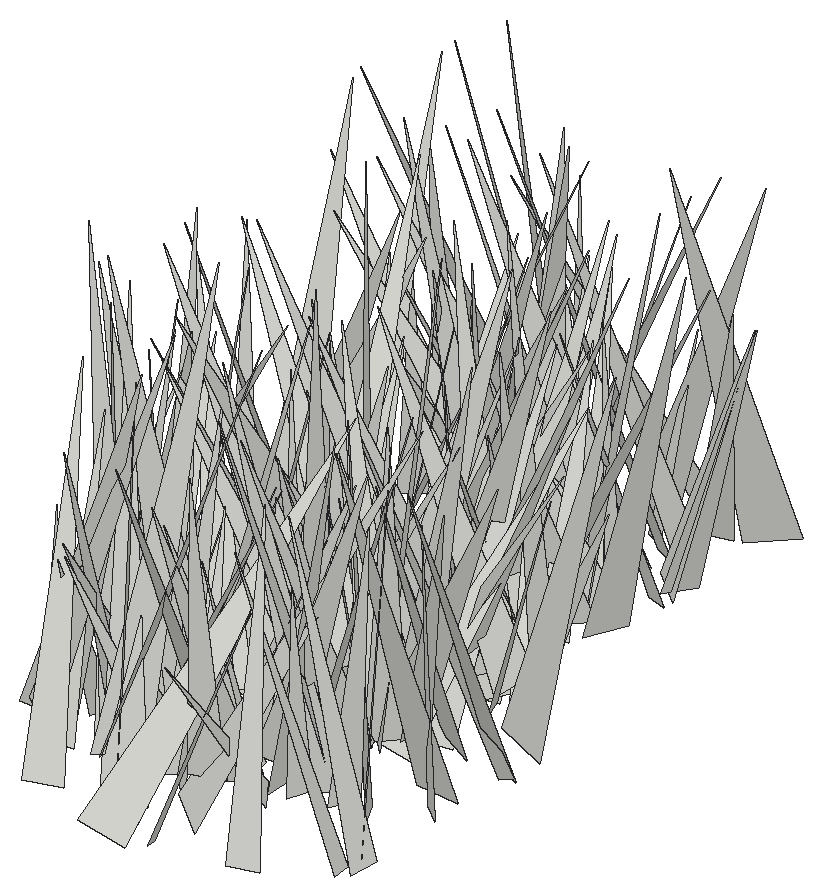
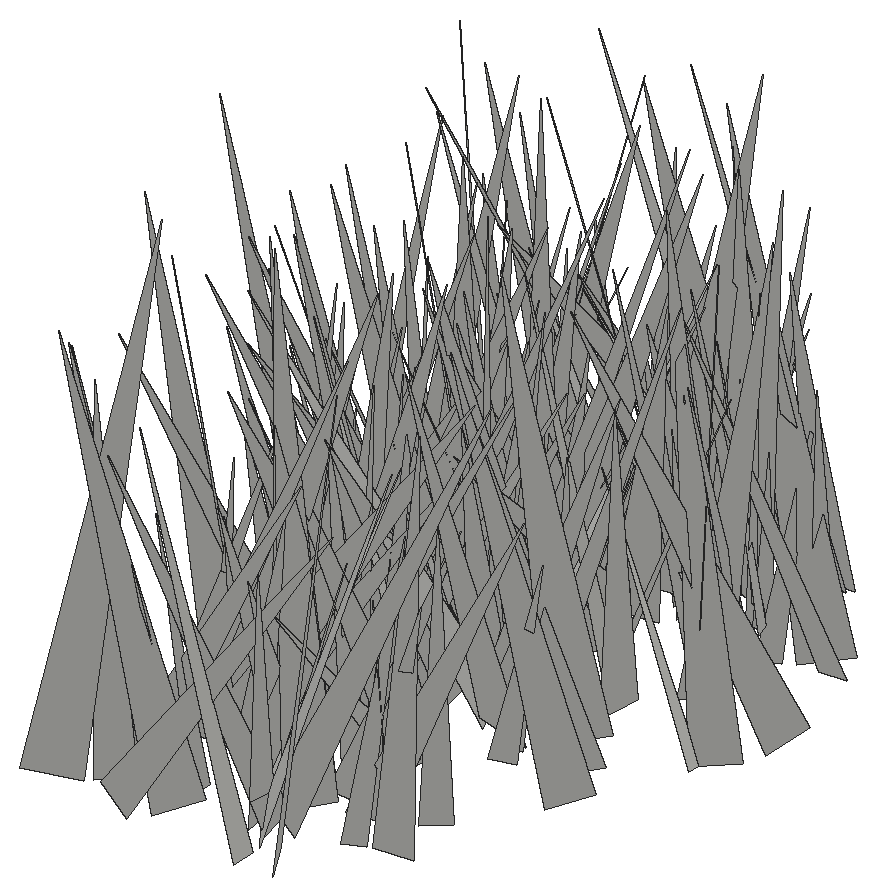
# SketchUp Ruby script. Lengths in inches.
U = 1.inch
M = Sketchup.active_model
def pt(a) = Geom::Point3d.new(a.map { |v| v * U })
def face(e, loops, mat)
  f = e.add_face(loops[0].map { |a| pt(a) })
  loops[1..].each { |l| e.add_face(l.map { |a| pt(a) }).erase! }
  f.material = f.back_material = mat if mat
  f
end
# faces: each face lists its corners as indices into pts; further lists are holes
def faces(e, pts, list, mat = nil) = list.each { |f| face(e, (f[0].is_a?(Array) ? f : [f]).map { |l| l.map { |i| pts[i] } }, mat) }
# xy, xz, yz: faces in a plane at the given z, y or x. An outline is a flat list of corners, or four numbers for a rectangle; further outlines are holes
def ring(l) = l.size == 4 ? [[l[0], l[1]], [l[2], l[1]], [l[2], l[3]], [l[0], l[3]]] : l.each_slice(2).to_a
def flat(e, list, mat, &to3) = list.each { |f| face(e, (f[0].is_a?(Array) ? f : [f]).map { |l| ring(l).map { |u, v| to3.(u, v) } }, mat) }
def xy(e, z, list, mat = nil) = flat(e, list, mat) { |x, y| [x, y, z] }
def xz(e, y, list, mat = nil) = flat(e, list, mat) { |x, z| [x, y, z] }
def yz(e, x, list, mat = nil) = flat(e, list, mat) { |y, z| [x, y, z] }
def lines(e, pts, list) = list.each { |a, b| e.add_line(pt(pts[a]), pt(pts[b])) }
# prism: a flat outline (further loops are holes) pulled along v
def prism(e, loops, v, mat = nil)
  f = face(e, loops, mat); d = Geom::Vector3d.new(v.map { |x| x * U })
  f.pushpull(f.normal.samedirection?(d) ? d.length : -d.length)
end
def box(e, o, s, mat = nil) = prism(e, [[o, [o[0] + s[0], o[1], o[2]], [o[0] + s[0], o[1] + s[1], o[2]], [o[0], o[1] + s[1], o[2]]]], [0, 0, s[2]], mat)
def at(x, y, z, deg = 0) = Geom::Transformation.translation(pt([x, y, z])) * Geom::Transformation.rotation(ORIGIN, Z_AXIS, deg.degrees)
def axes(o, x, y, z) = Geom::Transformation.new([*x, 0, *y, 0, *z, 0, *pt(o).to_a, 1])
def part(name) = M.definitions.add(name)
# library, detail: a bought-in or finely detailed component or shape, given as its bounding box
def library(name, o, s) = part(name).tap { |d| box(d.entities, o, s) }
def detail(e, o, s) = box(e.add_group.entities, o, s)
def put(e, d, t, mat = nil) = e.add_instance(d, t).tap { |i| i.material = mat if mat }
def group(e, t, mat = nil) = e.add_group.tap { |g| g.transformation = t; g.material = mat if mat }.entities
root = M.entities
c1 = part("fur_instance\#9")
p = [[0.8125,0,1.79],[0.67,-0.02,1.48],[0,-0.11,0],[0,0.11,0]]
faces(c1.entities,p,[[0,1,2,3]])
put(root,c1,axes([148.45,197.79,-28.22],[4.8815,3.3845,2.02519],[2.72156,-5.22275,2.16824],[-2.85471,0.80828,5.53015]))
put(root,c1,axes([148.84,203.19,-27.1],[-5.6137,1.8249,1.28834],[1.63706,5.7317,-0.98561],[1.51991,0.56669,5.82001]))
put(root,c1,axes([148.67,199.6,-28.22],[-6.28621,2.90163,2.83322],[3.4688,6.55463,0.9835],[2.10096,-2.14018,6.85337]))
put(root,c1,axes([150.45,212.51,-27.1],[-4.33976,4.07233,1.17149],[4.17045,3.80756,2.21352],[-0.75076,-2.38923,5.52429]))
put(root,c1,axes([148.03,194.95,-28.22],[-3.33469,1.40616,1.82105],[1.56398,3.73727,-0.02186],[1.68745,-0.685,3.61897]))
put(root,c1,axes([145.95,202.4375,-28.22],[2.99312,-6.69994,0.30324],[-6.59145,-2.87731,1.48788],[1.23852,0.87852,7.18569]))
put(root,c1,axes([146.57,196.35,-28.22],[1.84734,5.85191,0.92453],[5.8229,-1.61485,-1.41361],[1.09242,-1.28828,5.97153]))
put(root,c1,axes([146.28,202.97,-28.22],[4.26627,1.55205,0.05399],[1.49304,-4.05567,-1.39111],[0.42732,-1.32496,4.32143]))
put(root,c1,axes([145.1875,200.12,-28.22],[6.82569,-2.14516,0.01525],[-2.06759,-6.56497,1.95405],[0.57187,1.86856,6.88284]))
put(root,c1,axes([147.71,200.6,-28.22],[0.28341,4.29415,2.46111],[4.89058,0.13603,-0.80051],[0.76092,-2.47364,4.22839]))
put(root,c1,axes([149.52,207.61,-27.1],[-2.08975,2.94897,0.92989],[3.09202,1.98432,0.65582],[-0.0238,-1.13764,3.55435]))
put(root,c1,axes([150.25,195.58,-27.1],[-7.50799,1.69583,1.59774],[1.55933,7.66276,-0.80567],[1.73121,0.45255,7.65484]))
put(root,c1,axes([150.14,195.61,-28.22],[-6.12572,-2.31991,2.2614],[-2.97153,5.95041,-1.94497],[1.2907,2.68904,6.25488]))
put(root,c1,axes([148.5,196.86,-28.22],[3.04717,-2.22298,0.43436],[-2.028,-3.00193,-1.13631],[-1.00873,-0.67996,3.59662]))
put(root,c1,axes([148.62,213.68,-27.1],[0.4786,-6.17329,1.68247],[-6.39725,-0.42884,0.2463],[0.12453,1.69584,6.18692]))
put(root,c1,axes([150.45,204.91,-27.1],[-3.80657,-5.75041,0.9295],[-5.82495,3.76407,-0.56819],[0.03325,1.08891,6.87272]))
put(root,c1,axes([148.57,205.27,-27.1],[-4.94866,6.16749,2.69055],[6.18584,5.48419,-1.19385],[2.6481,-1.28527,7.81677]))
put(root,c1,axes([149.66,195.58,-28.22],[-0.46969,3.55211,0.73396],[3.59032,0.35011,0.60316],[-0.51554,-0.79795,3.53189]))
put(root,c1,axes([146.56,208.22,-27.1],[5.35038,-4.23141,0.69897],[-4.27634,-5.17862,1.38378],[0.32603,1.51562,6.67957]))
put(root,c1,axes([149.92,192.2,-28.22],[-1.0825,6.58238,0.66021],[6.6005,1.02978,0.55528],[-0.44383,-0.73975,6.64764]))
put(root,c1,axes([151.19,205.61,-27.1],[-5.49496,2.98551,0.84144],[3.09795,5.36781,1.18541],[0.15494,-1.44541,6.14025]))
put(root,c1,axes([148.7,211.6,-27.1],[2.93376,-3.22318,1.07266],[-3.3076,-3.03341,-0.06853],[-0.77414,0.74566,4.35788]))
put(root,c1,axes([149.74,202.73,-27.1],[-4.13984,-2.04423,0.54277],[-1.65039,3.86825,1.98107],[1.32277,-1.57147,4.17043]))
put(root,c1,axes([151.35,210.93,-27.1],[-1.53438,4.71255,0.03454],[4.47921,1.44703,1.55125],[-1.46492,-0.51147,4.70702]))
put(root,c1,axes([148.5,197.11,-27.1],[3.90059,1.73334,0.99556],[1.91928,-3.85762,-0.80331],[-0.55855,-1.15086,4.19211]))
put(root,c1,axes([152.39,214.02,-27.1],[-3.30387,-7.05223,0.96215],[-6.92829,2.9435,-2.21582],[-1.63048,1.78244,7.4659]))
put(root,c1,axes([150,192.89,-27.1],[0.07202,5.27236,0.64208],[5.29211,-0.12578,0.43929],[-0.45123,-0.63374,5.25452]))
put(root,c1,axes([149.73,196.04,-27.1],[1.82838,5.64567,1.15342],[5.69001,-1.95997,0.57384],[-0.90985,-0.91206,5.90655]))
put(root,c1,axes([150.57,206.29,-27.1],[0.71123,8.26754,0.30404],[8.18462,-0.74766,1.1847],[-1.20692,-0.19821,8.21307]))
put(root,c1,axes([152.47,214.85,-27.1],[-6.0406,-4.0795,1.11122],[-4.22494,5.74856,-1.86274],[-0.16426,2.16279,7.04708]))
put(root,c1,axes([149.84,206.84,-27.1],[0.38747,-3.62863,0.53891],[-3.66751,-0.39531,-0.02484],[-0.08219,0.53319,3.64917]))
put(root,c1,axes([150.79,197.07,-27.1],[-7.20595,2.28011,2.02761],[1.9171,7.42879,-1.54068],[2.37378,0.922,7.39939]))
put(root,c1,axes([150.32,197.63,-27.1],[-4.40906,-3.22075,2.19411],[-3.50304,4.72714,-0.10035],[1.70765,1.38134,5.45921]))
put(root,c1,axes([151.9,198.71,-27.1],[-2.77056,6.19265,0.76015],[6.19361,2.62958,1.15202],[-0.75223,-1.15721,6.68563]))
put(root,c1,axes([147.24,195.79,-28.22],[3.43501,-7.39782,1.03394],[-7.28345,-3.06455,2.27067],[1.65774,1.86463,7.83397]))
put(root,c1,axes([150.1,212.05,-27.1],[-2.43911,-2.15453,1.73505],[-2.51562,2.68975,-0.19638],[1.15067,1.31336,3.24849]))
put(root,c1,axes([150.4,196.83,-27.1],[-3.17134,4.85922,0.78552],[4.77597,3.26378,-0.90795],[1.19131,-0.14895,5.73106]))
put(root,c1,axes([150.9,216.07,-27.1],[-6.29622,-3.82649,2.40942],[-4.00808,6.63484,0.06324],[2.09347,1.19444,7.36752]))
put(root,c1,axes([149.81,213.97,-27.1],[4.21418,-1.38432,0.79636],[-0.98829,-4.02576,-1.76817],[-1.25452,-1.47878,4.06808]))
put(root,c1,axes([150.43,197.78,-28.22],[6.05789,3.57549,2.196],[3.19122,-6.43003,1.66595],[-2.72445,0.41853,6.83424]))
put(root,c1,axes([147.38,206.58,-27.1],[1.67696,-6.87357,2.26471],[-6.67493,-0.57073,3.21041],[2.79647,2.7596,6.30488]))
put(root,c1,axes([150.59,197.1,-28.22],[3.46816,-3.92613,0.03464],[-3.68547,-3.27126,-1.77763],[-1.35388,-1.15247,4.92774]))
put(root,c1,axes([150.375,196.96,-28.22],[3.62249,2.81644,0.55831],[2.6251,-3.61284,1.19278],[-1.16313,0.61769,4.43081]))
put(root,c1,axes([150.95,194.77,-27.1],[-1.08369,-5.40972,1.03151],[-5.49173,1.14023,0.21038],[0.41232,0.96864,5.51318]))
put(root,c1,axes([153.38,213.62,-27.1],[-5.70122,-3.26457,0.62497],[-3.32356,5.6155,-0.98593],[0.04408,1.16649,6.49533]))
put(root,c1,axes([148.5,193.81,-27.1],[4.58596,6.39713,1.96066],[6.63658,-4.04695,-2.31874],[0.85046,-2.91504,7.52182]))
put(root,c1,axes([152.2,201.56,-27.1],[0.68638,4.30492,0.85677],[4.11958,-0.93113,1.37825],[-1.51508,-0.58153,4.13569]))
put(root,c1,axes([152.6,192.77,-28.22],[-0.59735,8.07244,1.41711],[8.08686,0.34954,1.4177],[-1.33238,-1.49761,7.96939]))
put(root,c1,axes([152.82,202.95,-28.22],[-5.31992,-4.92486,0.01845],[-4.88394,5.27914,0.91325],[0.63384,-0.65774,7.19179]))
put(root,c1,axes([152.01,197.05,-27.1],[2.92408,-7.38877,2.72238],[-7.56214,-3.44459,-1.22649],[-2.19528,2.02396,7.85111]))
put(root,c1,axes([151.8,211.95,-27.1],[1.73038,-3.85975,0.19684],[-3.59553,-1.68683,-1.46882],[-1.41726,-0.43309,3.96667]))
put(root,c1,axes([150.76,204,-27.1],[2.98723,-2.64764,1.00912],[-2.72025,-3.09017,-0.05514],[-0.79284,0.62671,3.99131]))
put(root,c1,axes([152.11,194.84,-27.1],[-3.71284,-0.24914,0.82183],[0.046,3.58403,1.29433],[0.85753,-1.27095,3.48884]))
put(root,c1,axes([153.27,201.42,-27.1],[-6.87965,3.10007,2.46286],[3.78941,6.58637,2.29475],[1.14737,-3.16466,7.18848]))
put(root,c1,axes([153.77,200.68,-27.1],[-5.93019,0.58333,0.46706],[0.68124,5.75556,1.46115],[0.30714,-1.50292,5.77689]))
put(root,c1,axes([154.13,210.92,-27.1],[-6.77007,0.71674,0.61078],[0.8862,6.3486,2.37288],[0.31848,-2.42944,6.38099]))
put(root,c1,axes([151.22,194.29,-28.22],[5.6621,3.46946,2.68851],[3.90579,-5.98471,-0.5026],[-2.00251,-1.86297,6.62147]))
put(root,c1,axes([152.91,203.97,-27.1],[-5.36407,2.31527,0.60969],[2.0889,5.25672,-1.5839],[1.1699,1.22955,5.6236]))
put(root,c1,axes([150.23,201.83,-27.1],[5.73054,2.09287,1.0832],[2.24178,-5.71944,-0.8093],[-0.7265,-1.14039,6.04684]))
put(root,c1,axes([152.79,214.39,-27.1],[-4.924,0.48292,1.1816],[0.20052,4.94285,-1.18453],[1.26062,1.10005,4.80373]))
put(root,c1,axes([152.63,195.17,-28.22],[-5.40299,1.91129,1.15946],[1.49374,5.34299,-1.84687],[1.66317,1.41036,5.42535]))
put(root,c1,axes([152.04,198.8,-27.1],[-5.06896,3.36354,0.19703],[2.56301,4.08037,-3.71862],[2.18706,3.01393,4.81452]))
put(root,c1,axes([152.33,204.36,-27.1],[-7.59167,-1.95799,2.55179],[-0.44126,7.11339,4.14535],[3.18601,-3.68034,6.65457]))
put(root,c1,axes([152.76,214.125,-27.1],[-3.61548,-1.81279,0.7212],[-1.71327,3.67656,0.65243],[0.9333,-0.2734,3.99152]))
put(root,c1,axes([151.51,210.83,-27.1],[5.83634,-0.86723,1.56304],[-0.35494,-5.79341,-1.88904],[-1.75191,-1.71533,5.58985]))
put(root,c1,axes([152.27,209.05,-27.1],[3.66299,2.22216,0.32756],[1.7102,-3.16536,2.34915],[-1.4562,1.87225,3.58288]))
put(root,c1,axes([151.84,193.47,-27.1],[6.54564,-3.57049,3.76512],[-4.66006,-6.71077,1.73761],[-2.28219,3.46223,7.25083]))
put(root,c1,axes([152.76,203.82,-28.22],[-1.02276,3.4571,1.0392],[3.60758,1.01767,0.16502],[0.12981,-1.04418,3.60144]))
put(root,c1,axes([153.46,202.69,-28.22],[-6.14594,-1.15799,1.95321],[-1.28361,6.42082,-0.2323],[1.87305,0.60056,6.24977]))
put(root,c1,axes([152.98,201.9,-27.1],[-2.31741,7.72302,0.72504],[7.71845,2.37113,-0.58682],[0.77216,-0.52327,8.04183]))
put(root,c1,axes([153.93,202.93,-27.1],[-4.87029,1.64927,0.93909],[1.65484,4.95663,-0.12272],[0.92923,-0.18296,5.1405]))
put(root,c1,axes([153.1,195.9,-27.1],[-2.61192,2.51011,0.78878],[2.46687,2.72278,-0.49597],[0.91509,-0.17543,3.58843]))
put(root,c1,axes([153.75,201.96,-27.1],[-4.82421,0.67017,1.12309],[0.52178,4.9221,-0.69578],[1.19925,0.5543,4.82058]))
put(root,c1,axes([155.94,204.77,-28.22],[-4.22462,-4.77942,0.40733],[-4.62488,3.91455,-2.0354],[-1.27248,1.63999,6.04544]))
put(root,c1,axes([154.14,198.39,-28.22],[-4.53148,2.02632,0.31118],[1.79338,4.28391,-1.78018],[0.99329,1.50971,4.63371]))
put(root,c1,axes([157.59,209.46,-27.1],[-2.51256,7.06983,2.10699],[6.38069,0.96553,4.36915],[-3.70253,-3.13371,6.09968]))
put(root,c1,axes([153.18,204.625,-27.1],[3.77893,2.89431,1.05154],[2.64296,-3.90266,1.24382],[-1.58036,0.3941,4.59459]))
put(root,c1,axes([156.48,209.62,-27.1],[-2.71557,-5.16024,0.69315],[-4.67023,2.06855,-2.89705],[-2.30163,1.89099,5.06058]))
put(root,c1,axes([152.89,196.58,-27.1],[-1.67702,-6.45132,0.05531],[-6.32349,1.655,1.30744],[1.27907,-0.27646,6.53625]))
put(root,c1,axes([156.71,216.1875,-27.1],[-1.84266,-5.86998,0.99209],[-5.21002,1.08759,-3.24178],[-2.88039,1.78795,5.22904]))
put(root,c1,axes([151.29,209.36,-27.1],[5.01849,-2.22986,0.6447],[-2.32023,-4.77497,1.54574],[0.06662,1.67347,5.26955]))
put(root,c1,axes([153.2,209.5,-27.1],[-2.5079,-4.6968,1.95628],[-4.90602,2.8103,0.45782],[1.34828,1.48955,5.3047]))
put(root,c1,axes([154.33,211.01,-27.1],[-4.2837,1.86088,0.37109],[1.60299,4.03921,-1.75094],[1.01537,1.47394,4.32979]))
put(root,c1,axes([156.03,206.84,-27.1],[-0.49595,7.7495,2.67586],[7.77568,-0.40515,2.61451],[-2.59882,-2.6911,7.31198]))
put(root,c1,axes([156,203.66,-27.1],[-8.03194,-0.35365,0.82088],[-0.22203,7.97883,1.26494],[0.86581,-1.23463,7.93959]))
put(root,c1,axes([155.05,201.46,-27.1],[-7.31055,-2.64435,2.80127],[-3.45475,7.15889,-2.25809],[1.70424,3.16886,7.43894]))
put(root,c1,axes([155.22,211.83,-27.1],[-1.00856,5.27208,0.80529],[5.17147,0.76643,1.45913],[-1.30357,-1.0384,5.16556]))
put(root,c1,axes([154.18,204.07,-27.1],[-5.33853,3.8285,0.2094],[3.37353,4.86067,-2.86257],[1.82225,2.21756,5.91295]))
put(root,c1,axes([154.48,196.7,-28.22],[-4.67386,-0.0885,1.27111],[0.2568,4.66814,1.26925],[1.24804,-1.29194,4.49909]))
put(root,c1,axes([152.24,202.57,-28.22],[-2.5167,4.57974,3.46384],[4.9953,3.61127,-1.14527],[2.83182,-2.30014,5.09864]))
put(root,c1,axes([151.6,208.53,-27.1],[5.88028,2.97965,0.94292],[3.11911,-5.72141,-1.37172],[-0.19635,-1.65292,6.44782]))
put(root,c1,axes([153.51,211.98,-27.1],[-2.74828,4.07366,1.32335],[3.94461,3.01992,-1.10419],[1.66916,-0.42944,4.78838]))
put(root,c1,axes([151.08,194.02,-27.1],[7.89024,2.57718,0.73013],[2.64489,-7.85516,-0.85554],[-0.42369,-1.04189,8.25626]))
put(root,c1,axes([151.71,205.39,-27.1],[7.40987,3.38689,0.1989],[3.26816,-7.25381,1.76579],[-0.91088,1.52574,7.95356]))
put(root,c1,axes([152.37,192.49,-28.22],[5.57667,1.59527,0.3002],[1.43066,-5.3377,1.78788],[-0.76695,1.64269,5.51794]))
put(root,c1,axes([154.5625,196.15,-28.22],[1.51534,-5.37644,0.92666],[-5.31705,-1.67082,-0.99923],[-1.22223,0.60275,5.49581]))
put(root,c1,axes([155.57,195.81,-28.22],[-3.57996,-1.2077,0.30439],[-1.24532,3.48547,-0.8173],[0.0195,0.87192,3.68872]))
put(root,c1,axes([152.14,213.01,-27.1],[7.73764,-3.02475,0.93063],[-2.93122,-7.77665,-0.90436],[-1.19293,-0.51074,8.25847]))
put(root,c1,axes([151.74,216.54,-27.1],[6.21728,1.67139,0.47713],[1.73743,-6.02723,-1.52629],[-0.05031,-1.59834,6.25448]))
put(root,c1,axes([153.46,192.27,-28.22],[4.07971,3.91858,0.07723],[3.79656,-3.97882,1.32677],[-0.97331,0.90496,5.499]))
put(root,c1,axes([156.125,200.76,-27.1],[-1.77005,-3.87903,0.89181],[-3.77258,1.32393,-1.7292],[-1.26879,1.475,3.89741]))
put(root,c1,axes([157.04,213.35,-27.1],[-4.74845,-6.02691,1.04144],[-6.05438,4.44477,-1.88271],[-0.8676,1.96887,7.4382]))
put(root,c1,axes([153.15,212.03,-27.1],[4.39252,-6.51911,2.0007],[-6.79057,-4.39945,0.57342],[-0.62428,1.98542,7.83991]))
put(root,c1,axes([152.29,214.32,-27.1],[6.26365,0.83218,0.34032],[0.77044,-6.2027,0.98722],[-0.46342,0.93576,6.24109]))
put(root,c1,axes([157.69,213.69,-27.1],[-2.26256,-5.81888,2.33683],[-5.71547,0.89178,-3.31322],[-2.57945,3.12805,5.2916]))
put(root,c1,axes([152.9,195.02,-28.22],[5.81873,5.70667,1.51485],[5.84557,-5.86726,-0.35074],[-0.83073,-1.31442,8.14252]))
put(root,c1,axes([152.5,199.05,-28.22],[1.73127,-4.9492,1.56465],[-4.93445,-1.0575,2.11492],[1.61056,2.08017,4.79781]))
put(root,c1,axes([152.55,210.51,-27.1],[6.00758,0.21792,0.49644],[0.387,-5.59183,-2.22857],[-0.3797,-2.2514,5.58318]))
put(root,c1,axes([156.76,211.76,-27.1],[2.25381,-7.00366,2.80187],[-6.80723,-3.14832,-2.39397],[-3.25014,1.7373,6.957]))
put(root,c1,axes([152.66,208.02,-27.1],[7.35605,-1.97253,1.00478],[-2.03855,-7.39535,0.40615],[-0.86301,0.65556,7.60509]))
put(root,c1,axes([153.2,190.92,-28.22],[-3.48939,6.7058,0.49493],[5.71017,3.24965,-3.77124],[3.55058,1.36403,6.55144]))
put(root,c1,axes([155.49,197.87,-28.22],[-3.82053,1.38738,1.41647],[1.59253,3.97908,0.39802],[1.18113,-0.87734,4.0451]))
put(root,c1,axes([155.77,197.45,-27.1],[-5.23053,3.77379,0.03544],[3.44734,4.80229,-2.57973],[1.53577,2.07308,5.91142]))
put(root,c1,axes([154.62,200.27,-28.22],[4.44508,-4.04211,0.97735],[-3.87336,-4.54492,-1.18043],[-1.51359,-0.24009,5.89101]))
put(root,c1,axes([154.79,194.0625,-27.1],[1.69924,-5.28596,1.58911],[-5.50046,-1.7602,0.02657],[-0.46001,1.5213,5.5523]))
put(root,c1,axes([154.65,199.46,-27.1],[7.21029,-1.27081,2.71678],[-1.16788,-7.70491,-0.50453],[-2.76259,-0.05954,7.30402]))
put(root,c1,axes([152.83,208.0625,-27.1],[3.6305,3.98779,0.322],[3.84064,-3.3521,-1.78874],[1.12055,-1.43096,5.08758]))
put(root,c1,axes([157.1,203.86,-27.1],[2.35436,-6.19743,2.05043],[-5.78585,-2.99044,-2.39512],[-3.02263,0.89697,6.18179]))
put(root,c1,axes([155.08,201.26,-28.22],[3.76786,2.01641,1.4087],[2.07515,-3.9894,0.15999],[-1.32064,-0.51569,4.27049]))
put(root,c1,axes([154.77,191.39,-28.22],[4.06306,2.1594,0.43468],[1.91332,-3.91175,1.54848],[-1.0914,1.18135,4.33286]))
put(root,c1,axes([156.38,210.33,-27.1],[-4.08982,2.78235,0.32679],[2.66533,4.04258,-1.06229],[0.86271,0.7007,4.83111]))
put(root,c1,axes([156.14,200.41,-27.1],[-2.17091,-2.72609,1.07786],[-2.90812,2.17161,-0.36485],[0.36901,1.07644,3.46573]))
put(root,c1,axes([156.77,200.03,-27.1],[-4.49758,4.50366,1.60112],[4.72062,4.53017,0.51777],[0.74986,-1.50644,6.34374]))
put(root,c1,axes([153.26,201.75,-27.1],[3.75203,3.55416,0.24846],[3.4305,-3.50645,-1.64561],[0.96201,-1.35805,4.89916]))
put(root,c1,axes([155.6,195.92,-28.22],[-3.33896,-2.6162,0.26799],[-2.1089,2.92233,2.25332],[1.57125,-1.6372,3.59384]))
put(root,c1,axes([157.27,204.96,-28.22],[-6.9298,2.98954,1.57704],[3.02348,7.09089,-0.15622],[1.51094,-0.47802,7.54553]))
put(root,c1,axes([154.86,202.71,-27.1],[3.10305,4.72146,0.30771],[4.72969,-3.10544,-0.04628],[-0.13026,-0.28259,5.64969]))
put(root,c1,axes([156.55,203.99,-28.22],[-3.59286,-3.26733,2.03566],[-3.70516,3.69058,-0.61592],[1.04455,1.85261,4.81713]))
put(root,c1,axes([157.25,198.83,-27.1],[2.56501,3.25674,2.5986],[3.3721,-3.41499,0.95138],[-2.44704,-1.29222,4.03491]))
put(root,c1,axes([155.16,214.19,-27.1],[4.1341,0.32333,0.78637],[0.3951,-4.18703,-0.35553],[-0.75288,-0.42186,4.13146]))
put(root,c1,axes([154.35,195.75,-27.1],[4.46845,1.48023,0.19389],[1.49287,-4.43008,-0.58427],[0.00126,-0.6156,4.67084]))
put(root,c1,axes([158.12,195.58,-27.1],[-0.65544,-6.57541,2.82853],[-6.91722,-0.14862,-1.94837],[-1.84083,2.89967,6.31422]))
put(root,c1,axes([155.66,207.92,-27.1],[4.05773,-0.76512,0.97615],[-0.40955,-3.97873,-1.41614],[-1.1707,-1.26007,3.87881]))
put(root,c1,axes([156.83,204.53,-28.22],[-6.41092,4.00729,0.82453],[3.32918,6.00061,-3.27831],[2.37798,2.40258,6.81256]))
put(root,c1,axes([154.23,203.48,-28.22],[8.0865,0.10169,1.15451],[-0.2162,-7.86244,2.20681],[-1.13864,2.21504,7.78021]))
put(root,c1,axes([156.18,213.92,-27.1],[1.71748,3.11444,0.84575],[3.20742,-1.75327,-0.057],[-0.35706,-0.7688,3.55615]))
put(root,c1,axes([154.86,203.34,-27.1],[3.44666,-5.98968,2.82803],[-6.61551,-2.95389,1.80641],[0.33028,3.33943,6.67028]))
put(root,c1,axes([157.67,198.08,-27.1],[-5.8236,-1.97497,1.08531],[-1.72724,5.8434,1.36532],[1.44743,-0.9731,5.99589]))
put(root,c1,axes([156.77,202.31,-28.22],[0.14678,4.73777,0.12743],[4.7339,-0.15274,0.22615],[-0.23006,-0.12022,4.73465]))
put(root,c1,axes([158.5,204.25,-27.1],[-6.51837,1.52305,1.37348],[1.82295,6.39951,1.5551],[0.93967,-1.84981,6.5108]))
put(root,c1,axes([156.52,206.8,-27.1],[-1.70648,-4.83175,0.15849],[-4.67215,1.69151,1.26205],[1.24174,-0.27565,4.96639]))
put(root,c1,axes([156.48,207.24,-27.1],[5.03393,-2.19184,1.50174],[-1.99616,-5.24318,-0.96135],[-1.75349,-0.32355,5.40559]))
put(root,c1,axes([157.84,196.5625,-27.1],[-5.81163,-3.8947,1.27527],[-3.71182,5.94036,1.22659],[1.73708,-0.33677,6.88761]))
put(root,c1,axes([157.57,208.48,-27.1],[1.87791,-4.76016,0.94457],[-4.63856,-2.05833,-1.15104],[-1.42657,0.4266,4.98606]))
put(root,c1,axes([158.76,205.38,-27.1],[-7.01031,-0.43579,1.43561],[-0.72042,6.99511,-1.39453],[1.31601,1.50792,6.88401]))
put(root,c1,axes([157.92,191.86,-28.22],[-0.40963,5.6712,0.85204],[5.69515,0.30195,0.72827],[-0.67361,-0.89587,5.63914]))
put(root,c1,axes([156.89,198.04,-27.1],[-2.21972,3.26489,1.22418],[3.2229,2.47495,-0.75684],[1.3308,-0.54808,3.87477]))
put(root,c1,axes([157.48,198.92,-27.1],[5.31201,5.41879,2.20999],[5.24419,-5.73235,1.45032],[-2.59727,-0.49162,7.44831]))
put(root,c1,axes([156.16,202.44,-27.1],[5.31281,-2.73186,1.51927],[-2.91837,-5.40827,0.48055],[-1.11999,1.13346,5.95467]))
put(root,c1,axes([157.54,201.49,-28.22],[-4.8564,4.18897,0.42907],[3.70643,4.56321,-2.59917],[1.99849,1.71635,5.86314]))
put(root,c1,axes([160.65,201.18,-28.22],[-3.53185,-5.19128,1.06072],[-4.89285,2.7062,-3.04713],[-2.03336,2.50511,5.48984]))
put(root,c1,axes([157.6,207.19,-27.1],[-2.09366,4.25191,0.8072],[4.26644,2.17826,-0.40798],[0.72654,-0.53866,4.72184]))
put(root,c1,axes([158.64,210.96,-27.1],[-2.25031,-4.2676,0.76277],[-4.32128,2.13921,-0.77999],[-0.34742,1.03417,4.76108]))
put(root,c1,axes([158.38,209.3,-27.1],[0.93593,4.40998,1.37185],[4.37962,-1.29175,1.16453],[-1.46587,-1.0437,4.3552]))
put(root,c1,axes([155.0625,205.12,-28.22],[6.11915,-4.70581,1.11272],[-4.83462,-5.98952,1.25659],[-0.09634,1.67568,7.61641]))
put(root,c1,axes([155.01,215.37,-27.1],[6.03076,-3.95506,0.64167],[-4.00583,-5.92637,1.12057],[0.08689,1.28836,7.12438]))
put(root,c1,axes([154.46,193.49,-28.22],[4.68977,6.59581,0.10077],[6.41242,-4.52929,-1.96857],[1.54784,-1.22048,7.85006]))
put(root,c1,axes([158.58,204.58,-28.22],[-2.11834,3.44874,0.2067],[3.45458,2.11778,0.0692],[0.04913,-0.21236,4.04678]))
put(root,c1,axes([156.87,195.06,-27.1],[6.13024,0.22864,1.74835],[0.20896,-6.37456,0.10097],[-1.75081,0.03976,6.13367]))
put(root,c1,axes([156.09,203.63,-28.22],[7.47336,0.82298,1.26079],[0.38429,-7.21504,2.43175],[-1.45575,2.3203,7.11442]))
put(root,c1,axes([157.63,194.99,-27.1],[3.35457,-1.66316,1.27005],[-1.64462,-3.57909,-0.343],[-1.29397,0.23728,3.72849]))
put(root,c1,axes([158.78,196.86,-28.22],[-5.34444,-2.84039,2.21318],[-3.30562,5.4408,-0.99979],[1.42788,1.96442,5.96919]))
put(root,c1,axes([160.32,193.62,-28.22],[-4.94313,-1.68267,0.02369],[-1.64372,4.81198,-1.18726],[-0.36076,1.13137,5.08492]))
put(root,c1,axes([156.68,209.86,-27.1],[-3.91032,-4.73518,3.93684],[-5.20514,5.03349,0.88414],[3.29046,2.33522,6.07707]))
put(root,c1,axes([157.58,199.1875,-27.1],[-3.8078,3.44308,3.43375],[4.19662,4.52997,0.11149],[2.45637,-2.40193,5.13242]))
put(root,c1,axes([156.82,200.4,-28.22],[-2.23637,5.81255,0.47787],[5.16217,2.21098,-2.73477],[2.71405,0.58421,5.59536]))
put(root,c1,axes([155.875,196.05,-27.1],[2.64878,-6.42579,1.07864],[-6.29914,-2.22772,2.19734],[1.66585,1.79353,6.59382]))
put(root,c1,axes([156.875,196.25,-27.1],[6.30339,2.19635,1.13005],[2.22882,-6.39265,-0.00763],[-1.06457,-0.37914,6.67507]))
put(root,c1,axes([156.54,207.65,-27.1],[6.37696,0.70596,0.43543],[0.57496,-6.19552,1.62437],[-0.59783,1.57187,6.20688]))
put(root,c1,axes([158.16,201.77,-28.22],[-1.98153,-6.18192,0.39554],[-6.00617,2.01899,1.46585],[1.5161,-0.08133,6.32408]))
put(root,c1,axes([155.1875,203.62,-28.22],[5.8756,3.65861,0.2575],[3.32747,-5.11292,-3.2803],[1.54262,-2.90637,6.0949]))
put(root,c1,axes([160.73,194.2,-28.22],[-5.68888,-0.08485,0.69236],[-0.12916,5.71868,-0.36046],[0.68548,0.37338,5.67808]))
put(root,c1,axes([157.1,203,-27.1],[5.55155,-0.72144,0.45458],[-0.77671,-5.51397,0.73462],[-0.35191,0.78896,5.54982]))
put(root,c1,axes([157.43,215.2,-27.1],[2.80299,-5.03768,0.10257],[-5.00094,-2.76705,0.76127],[0.6159,0.45904,5.71449]))
put(root,c1,axes([159.01,216.11,-27.1],[4.03591,-7.21522,0.98619],[-7.10178,-4.1491,-1.2924],[-1.61145,0.21471,8.16564]))
put(root,c1,axes([158.07,200.05,-27.1],[4.83385,-1.43847,0.54232],[-1.36908,-4.84202,-0.64023],[-0.69925,-0.46374,5.00254]))
put(root,c1,axes([156.54,201.91,-27.1],[0.60809,-6.43634,0.77652],[-5.71222,-0.16309,3.1214],[3.06594,0.97271,5.66154]))
put(root,c1,axes([159.02,195.38,-27.1],[4.44334,-1.86269,1.64457],[-2.02269,-4.66849,0.17731],[-1.44323,0.80817,4.81471]))
put(root,c1,axes([159.61,199.15,-28.22],[-0.40558,-7.48594,0.6627],[-7.51279,0.42075,0.15485],[0.19107,0.65318,7.49532]))
put(root,c1,axes([158.91,202.67,-27.1],[3.66327,1.41122,0.72087],[1.44956,-3.71776,-0.08822],[-0.64027,-0.34277,3.92471]))
put(root,c1,axes([160.22,198.09,-28.22],[-3.07714,-3.38347,1.94932],[-3.73457,3.27489,-0.21099],[1.14047,1.59489,4.5686]))
put(root,c1,axes([158.33,211.84,-27.1],[3.55889,4.26793,1.49162],[4.48448,-3.09137,-1.85436],[0.57409,-2.30955,5.23854]))
put(root,c1,axes([158.59,208.58,-27.1],[6.87118,-2.4682,1.14103],[-2.53265,-6.93781,0.24398],[-0.98977,0.61792,7.29696]))
put(root,c1,axes([158.73,211.97,-27.1],[5.12871,-2.48578,0.55768],[-2.53054,-5.11559,0.47007],[-0.29413,0.66743,5.67995]))
put(root,c1,axes([160.08,201.68,-28.22],[-2.24137,-6.8028,0.2078],[-6.58087,2.22202,1.76064],[1.73594,-0.35988,6.94277]))
put(root,c1,axes([158.97,204.54,-27.1],[2.19638,-3.75423,0.49776],[-3.62923,-1.92217,1.51658],[1.08198,1.1735,4.07656]))
put(root,c1,axes([159.93,195.09,-28.22],[-5.21121,-4.35385,3.58957],[-4.50193,6.15376,0.92827],[3.40202,1.4741,6.72689]))
put(root,c1,axes([159.71,203.04,-28.22],[2.12208,6.92928,3.4126],[7.54208,-1.09525,-2.46604],[1.66665,-3.86645,6.81445]))
